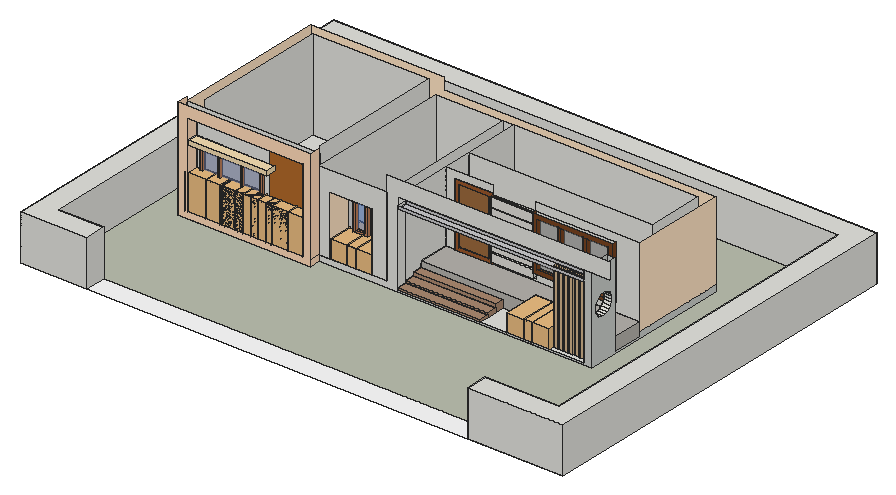
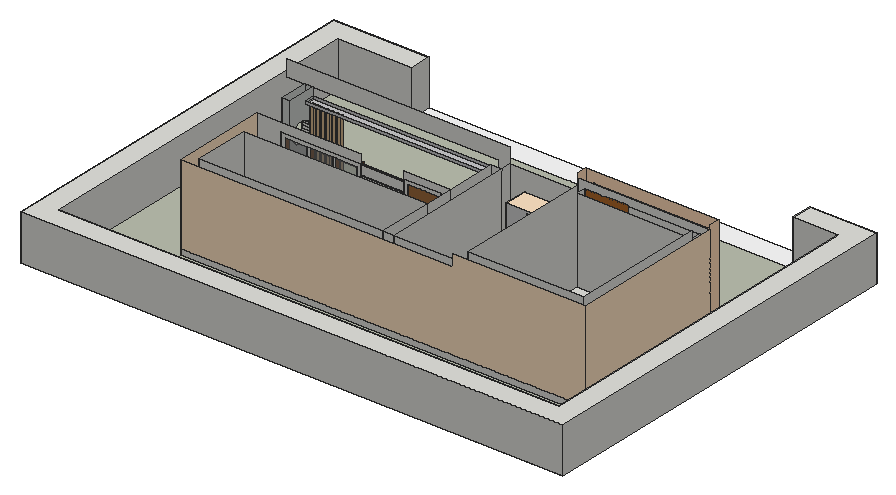
# SketchUp Ruby script. Lengths in inches.
U = 1.inch
M = Sketchup.active_model
def pt(a) = Geom::Point3d.new(a.map { |v| v * U })
def face(e, loops, mat)
  f = e.add_face(loops[0].map { |a| pt(a) })
  loops[1..].each { |l| e.add_face(l.map { |a| pt(a) }).erase! }
  f.material = f.back_material = mat if mat
  f
end
# faces: each face lists its corners as indices into pts; further lists are holes
def faces(e, pts, list, mat = nil) = list.each { |f| face(e, (f[0].is_a?(Array) ? f : [f]).map { |l| l.map { |i| pts[i] } }, mat) }
# xy, xz, yz: faces in a plane at the given z, y or x. An outline is a flat list of corners, or four numbers for a rectangle; further outlines are holes
def ring(l) = l.size == 4 ? [[l[0], l[1]], [l[2], l[1]], [l[2], l[3]], [l[0], l[3]]] : l.each_slice(2).to_a
def flat(e, list, mat, &to3) = list.each { |f| face(e, (f[0].is_a?(Array) ? f : [f]).map { |l| ring(l).map { |u, v| to3.(u, v) } }, mat) }
def xy(e, z, list, mat = nil) = flat(e, list, mat) { |x, y| [x, y, z] }
def xz(e, y, list, mat = nil) = flat(e, list, mat) { |x, z| [x, y, z] }
def yz(e, x, list, mat = nil) = flat(e, list, mat) { |y, z| [x, y, z] }
def lines(e, pts, list) = list.each { |a, b| e.add_line(pt(pts[a]), pt(pts[b])) }
# prism: a flat outline (further loops are holes) pulled along v
def prism(e, loops, v, mat = nil)
  f = face(e, loops, mat); d = Geom::Vector3d.new(v.map { |x| x * U })
  f.pushpull(f.normal.samedirection?(d) ? d.length : -d.length)
end
def box(e, o, s, mat = nil) = prism(e, [[o, [o[0] + s[0], o[1], o[2]], [o[0] + s[0], o[1] + s[1], o[2]], [o[0], o[1] + s[1], o[2]]]], [0, 0, s[2]], mat)
def at(x, y, z, deg = 0) = Geom::Transformation.translation(pt([x, y, z])) * Geom::Transformation.rotation(ORIGIN, Z_AXIS, deg.degrees)
def axes(o, x, y, z) = Geom::Transformation.new([*x, 0, *y, 0, *z, 0, *pt(o).to_a, 1])
def part(name) = M.definitions.add(name)
# library, detail: a bought-in or finely detailed component or shape, given as its bounding box
def library(name, o, s) = part(name).tap { |d| box(d.entities, o, s) }
def detail(e, o, s) = box(e.add_group.entities, o, s)
def put(e, d, t, mat = nil) = e.add_instance(d, t).tap { |i| i.material = mat if mat }
def group(e, t, mat = nil) = e.add_group.tap { |g| g.transformation = t; g.material = mat if mat }.entities
root = M.entities
M.materials.add("[0012_Bisque]").color = [255, 228, 196]
M.materials.add("[0027_PeachPuff]").color = [255, 218, 185]
M.materials.add("[0034_Wheat]").color = [245, 222, 179]
M.materials.add("[0035_Tan]").color = [210, 180, 140]
M.materials.add("[Basic Tile]").color = [203, 206, 202]
M.materials.add("[Cladding Siding White]").color = [207, 207, 207]
M.materials.add("[Color M00]").color = [255, 255, 255]
M.materials.add("[Pavers with Grass Brick]").color = [187, 192, 176]
M.materials.add("[Polished Concrete New]").color = [200, 200, 203]
M.materials.add("[Terrazzo Tile Accent]").color = [224, 221, 217]
M.materials.add("[Tile Travertine 2 inch]").color = [181, 178, 172]
M.materials.add("[Tile Veriegated Stone]").color = [171, 137, 112]
M.materials.add("[Translucent Glass Blue]").color = [100, 149, 237]
M.materials["[Translucent Glass Blue]"].alpha = 0.5
M.materials.add("[Translucent Glass Gray]").color = [128, 128, 128]
M.materials["[Translucent Glass Gray]"].alpha = 0.5
M.materials.add("[Translucent Glass Sky Reflection]").color = [126, 138, 183]
M.materials["[Translucent Glass Sky Reflection]"].alpha = 0.52
M.materials.add("[Wood Bamboo]").color = [177, 105, 43]
M.materials.add("[Wood Cherry Original]").color = [119, 67, 33]
M.materials.add("[Wood Cherry Original]1").color = [152, 86, 42]
M.materials.add("[Wood Floor]").color = [155, 105, 61]
M.materials.add("[Wood Veneer 02]").color = [190, 128, 91]
c1 = library("Flora+17",[-57.52,158.6,-38.64],[66.99,62.88,77.28])
c2 = library("chau cay",[-24.34,-109.24,0],[56.46,62.58,79.69])
xy(root,0,[[0,0,0,591.67,820.1875,591.67,820.1875,0,676.89,0,676.89,32.2,787.99,32.2,787.99,559.47,32.2,559.47,32.2,32.2,99.92,32.2,99.92,0],[72.24,206.91,272.73,223.85],[72.24,223.85,684.44,458.94]])
xy(root,0,[[99.92,0,676.89,32.2]],"[Color M00]")
xy(root,0,[[[32.2,32.2,787.99,559.47],[72.24,206.91,272.73,223.85]]],"[Pavers with Grass Brick]")
xy(root,2.375,[[391.12,223.85,515.24,238.73],[[515.24,223.85,671.95,268.03],[620.18,231.6,626.53,236.51],[628.05,231.6,634.31,236.51],[660.62,231.6,666.86,236.51],[643.87,231.6,649.89,236.51],[635.99,231.6,641.99,236.51],[652.18,231.6,658.09,236.51]],[620.18,231.6,626.53,236.51],[628.05,231.6,634.31,236.51],[635.99,231.6,641.99,236.51],
  [643.87,231.6,649.89,236.51],[652.18,231.6,658.09,236.51],[660.62,231.6,666.86,236.51],[391.12,238.73,515.24,253.38],[391.12,253.38,515.24,268.03]])
xy(root,5.8125,[[391.12,223.85,515.24,238.73]],"[Tile Veriegated Stone]")
xy(root,9,[[87.11,223.85,261.95,238.73],[272.73,223.85,272.73,444.0625,374.48,444.0625,374.48,223.85,352.6,223.85,352.6,259.48,287.9,259.48,287.9,223.85],[87.11,238.73,261.95,444.0625],[374.48,238.73,391.12,444.0625],[391.12,358.92,668.6875,444.0625]])
xy(root,9,[[287.9,223.85,352.6,259.48]],"[0012_Bisque]")
xy(root,9,[[87.11,206.91,261.95,223.85]],"[0027_PeachPuff]")
xy(root,9,[[391.12,238.73,515.24,253.38]],"[Tile Veriegated Stone]")
xy(root,14,[[391.12,253.38,515.24,268.03]],"[Tile Veriegated Stone]")
xy(root,22.51,[[406.1,313.78,461.1,315.41]])
xy(root,22.51,[[391.12,268.03,684.44,268.03,684.44,315.41,461.1,315.41,461.1,313.78,406.1,313.78,406.1,315.41,391.12,315.41]],"[Tile Travertine 2 inch]")
xy(root,26.45,[[461.1,311.53,526.2,315.41]],"[Terrazzo Tile Accent]")
xy(root,27.37,[[410.96,313.78,456.24,315.41]],"[Wood Cherry Original]1")
xy(root,34.36,[[298.82,254.6,320.82,259.48]],"[Wood Veneer 02]")
xy(root,34.89,[[526.2,309.72,646.95,315.41]])
xy(root,38.29,[[302.75,254.6,316.89,259.48]],"[Wood Veneer 02]")
xy(root,39.1875,[[461.1,311.53,526.2,315.41]])
xy(root,41.13,[[564.27,309.72,569.69,315.41],[602.52,309.72,607.94,315.41]])
xy(root,41.13,[[532.4375,309.72,564.27,315.41],[569.69,309.72,602.52,315.41],[607.94,309.72,640.71,315.41]],"[Wood Cherry Original]")
xy(root,41.89,[[461.1,311.53,526.2,315.41]],"[Terrazzo Tile Accent]")
xy(root,44.5,[[94.34,221.35,188.94,223.85]])
xy(root,48.77,[[121.4,221.35,124.96,223.85],[155.64,221.35,158.77,223.85]])
xy(root,48.77,[[98.6,221.35,121.4,223.85],[124.96,221.35,155.64,223.85],[158.77,221.35,184.67,223.85]],"[Wood Veneer 02]")
xy(root,54.625,[[461.1,311.53,526.2,315.41]])
xy(root,56.76,[[461.1,311.53,526.2,315.41]],"[Terrazzo Tile Accent]")
xy(root,69.1875,[[0,0,99.92,0,99.92,32.2,32.2,32.2,32.2,559.47,787.99,559.47,787.99,32.2,676.89,32.2,676.89,0,820.1875,0,820.1875,591.67,0,591.67]])
xy(root,69.5,[[461.1,311.53,526.2,315.41]])
xy(root,71.64,[[461.1,311.53,526.2,315.41]],"[Terrazzo Tile Accent]")
xy(root,84.375,[[461.1,311.53,526.2,315.41]])
xy(root,86.51,[[461.1,311.53,526.2,315.41]],"[Terrazzo Tile Accent]")
xy(root,92.31,[[302.75,254.6,316.89,259.48]])
xy(root,93.36,[[121.4,221.35,124.96,223.85],[155.64,221.35,158.77,223.85]])
xy(root,93.36,[[98.6,221.35,121.4,223.85],[124.96,221.35,155.64,223.85],[158.77,221.35,184.67,223.85]],"[Wood Veneer 02]")
xy(root,96.24,[[298.82,254.6,320.82,259.48]],"[Wood Veneer 02]")
xy(root,97.625,[[94.34,221.35,188.94,223.85]])
xy(root,99.25,[[461.1,311.53,526.2,315.41]])
xy(root,99.28,[[287.9,223.85,352.6,259.48]],"[0012_Bisque]")
xy(root,99.28,[[87.11,207.66,205.99,223.85]],"[0034_Wheat]")
xy(root,101.39,[[461.1,311.53,526.2,315.41]],"[Terrazzo Tile Accent]")
xy(root,105.41,[[87.11,207.66,205.99,223.85]],"[0034_Wheat]")
xy(root,110.47,[[564.27,309.72,569.69,315.41],[602.52,309.72,607.94,315.41]])
xy(root,110.47,[[532.4375,309.72,564.27,315.41],[569.69,309.72,602.52,315.41],[607.94,309.72,640.71,315.41]],"[Wood Cherry Original]")
xy(root,112.27,[[[391.12,223.85,671.95,238.73],[620.18,231.6,626.53,236.51],[628.05,231.6,634.31,236.51],[660.62,231.6,666.86,236.51],[643.87,231.6,649.89,236.51],[635.99,231.6,641.99,236.51],[652.18,231.6,658.09,236.51]]],"[Polished Concrete New]")
xy(root,113.71,[[410.96,313.78,456.24,315.41]],"[Wood Cherry Original]1")
xy(root,114.125,[[461.1,311.53,526.2,315.41]])
xz(root,0,[[0,0,99.92,69.1875],[676.89,0,820.1875,69.1875]])
xz(root,32.2,[[32.2,0,99.92,69.1875],[676.89,0,787.99,69.1875]])
xz(root,206.91,[[[72.24,0,272.73,152.4375],[87.11,9,261.95,135.55]]],"[0027_PeachPuff]")
xz(root,207.66,[[87.11,99.28,205.99,105.41]],"[0034_Wheat]")
xz(root,221.35,[[[94.34,44.5,188.94,97.625],[98.6,48.77,184.67,93.36]],[121.4,48.77,124.96,93.36],[155.64,48.77,158.77,93.36]],"[Wood Veneer 02]")
xz(root,223.85,[[[72.24,0,272.73,146.125],[87.11,9,261.95,135.55]],[272.73,0,391.12,0,391.12,129,711.13,129,711.13,152.4375,374.48,152.4375,374.48,9,272.73,9],[[87.11,9,196.88,99.28],[94.34,44.5,188.94,97.625]],[272.73,9,287.9,9,287.9,99.28,352.6,99.28,352.6,9,374.48,9,374.48,129,272.73,129],[[94.34,44.5,188.94,97.625],[98.6,48.77,184.67,93.36]],
  [121.4,48.77,124.96,93.36],[155.64,48.77,158.77,93.36],[87.11,99.28,196.88,105.41],[196.88,99.28,205.99,105.41],[87.11,105.41,196.88,135.55]])
xz(root,223.85,[[391.12,0,684.44,0,684.44,129,671.95,129,671.95,2.375,391.12,2.375]],"[Basic Tile]")
xz(root,223.85,[[391.12,112.27,671.95,116.34]],"[Polished Concrete New]")
xz(root,223.85,[[391.12,2.375,515.24,5.8125]],"[Tile Veriegated Stone]")
xz(root,223.85,[[98.6,48.77,121.4,93.36],[124.96,48.77,155.64,93.36],[158.77,48.77,184.67,93.36]],"[Translucent Glass Sky Reflection]")
xz(root,223.85,[[196.88,9,261.95,9,261.95,135.55,196.88,135.55,196.88,105.41,205.99,105.41,205.99,99.28,196.88,99.28]],"[Wood Bamboo]")
xz(root,231.6,[[620.18,2.375,626.53,112.27],[628.05,2.375,634.31,112.27],[635.99,2.375,641.99,112.27],[643.87,2.375,649.89,112.27],[652.18,2.375,658.09,112.27],
  [660.62,2.375,666.86,112.27]],"[0035_Tan]")
xz(root,236.51,[[620.18,2.375,626.53,112.27],[628.05,2.375,634.31,112.27],[635.99,2.375,641.99,112.27],[643.87,2.375,649.89,112.27],[652.18,2.375,658.09,112.27],
  [660.62,2.375,666.86,112.27]],"[0035_Tan]")
xz(root,238.73,[[391.12,2.375,515.24,5.8125],[87.11,9,261.95,135.55],[374.48,9,391.12,129]])
xz(root,238.73,[[391.12,112.27,671.95,116.34]],"[Polished Concrete New]")
xz(root,238.73,[[391.12,5.8125,515.24,9]],"[Tile Veriegated Stone]")
xz(root,253.38,[[391.12,2.375,515.24,9]])
xz(root,253.38,[[391.12,9,515.24,14]],"[Tile Veriegated Stone]")
xz(root,254.6,[[[298.82,34.36,320.82,96.24],[302.75,38.29,316.89,92.31]]],"[Wood Veneer 02]")
xz(root,259.48,[[[298.82,34.36,320.82,96.24],[302.75,38.29,316.89,92.31]]])
xz(root,259.48,[[[287.9,9,352.6,99.28],[298.82,34.36,320.82,96.24]]],"[Cladding Siding White]")
xz(root,259.48,[[302.75,38.29,316.89,92.31]],"[Translucent Glass Blue]")
xz(root,268.03,[[391.12,2.375,515.24,14]])
xz(root,268.03,[[671.95,22.51,684.44,129]],"[Basic Tile]")
xz(root,268.03,[[515.24,2.375,671.95,2.375,671.95,22.51,391.12,22.51,391.12,14,515.24,14]],"[Tile Travertine 2 inch]")
xz(root,309.72,[[[526.2,34.89,646.95,116.71],[532.4375,41.13,640.71,110.47]],[564.27,41.13,569.69,110.47],[602.52,41.13,607.94,110.47]],"[Wood Cherry Original]")
xz(root,311.53,[[461.1,26.45,526.2,39.1875],[461.1,41.89,526.2,54.625],[461.1,56.76,526.2,69.5],[461.1,71.64,526.2,84.375],[461.1,86.51,526.2,99.25],
  [461.1,101.39,526.2,114.125]],"[Terrazzo Tile Accent]")
xz(root,313.78,[[[406.1,22.51,461.1,118.57],[410.96,27.37,456.24,113.71]]],"[Wood Cherry Original]1")
xz(root,315.41,[[391.12,2.375,684.44,22.51],[391.12,22.51,406.1,22.51,406.1,118.57,461.1,118.57,461.1,129,391.12,129],[[406.1,22.51,461.1,118.57],[410.96,27.37,456.24,113.71]],[461.1,22.51,526.2,26.45],[526.2,22.51,684.44,22.51,684.44,129,526.2,129,526.2,116.71,646.95,116.71,646.95,34.89,526.2,34.89],
  [461.1,26.45,526.2,39.1875],[[526.2,34.89,646.95,116.71],[532.4375,41.13,640.71,110.47]],[461.1,39.1875,526.2,41.89],[564.27,41.13,569.69,110.47],[602.52,41.13,607.94,110.47],
  [461.1,41.89,526.2,54.625],[461.1,54.625,526.2,56.76],[461.1,56.76,526.2,69.5],[461.1,69.5,526.2,71.64],[461.1,71.64,526.2,84.375],
  [461.1,84.375,526.2,86.51],[461.1,86.51,526.2,99.25],[461.1,99.25,526.2,101.39],[461.1,101.39,526.2,114.125],[461.1,114.125,526.2,116.26]])
xz(root,315.41,[[532.4375,41.13,564.27,110.47],[569.69,41.13,602.52,110.47],[607.94,41.13,640.71,110.47]],"[Translucent Glass Gray]")
xz(root,315.41,[[410.96,27.37,456.24,113.71]],"[Wood Floor]")
xz(root,358.92,[[391.12,9,668.6875,129]])
xz(root,444.0625,[[87.11,9,261.95,146.125],[272.73,9,374.48,129],[374.48,9,391.12,129],[391.12,9,668.6875,129]])
xz(root,458.94,[[72.24,0,684.44,9]])
xz(root,458.94,[[72.24,9,72.24,146.125,272.73,146.125,272.73,129,684.44,129,684.44,9]],"[0012_Bisque]")
xz(root,559.47,[[32.2,0,787.99,69.1875]])
xz(root,591.67,[[0,0,820.1875,69.1875]])
yz(root,0,[[0,0,591.67,69.1875]])
yz(root,32.2,[[32.2,0,559.47,69.1875]])
yz(root,72.24,[[223.85,0,458.94,9]])
yz(root,72.24,[[223.85,9,458.94,146.125]],"[0012_Bisque]")
yz(root,72.24,[[206.91,0,223.85,9],[206.91,9,223.85,152.4375]],"[0027_PeachPuff]")
yz(root,87.11,[[223.85,9,238.73,135.55],[238.73,9,444.0625,146.125],[207.66,99.28,223.85,105.41]])
yz(root,87.11,[[206.91,9,223.85,9,223.85,99.28,207.66,99.28,207.66,105.41,223.85,105.41,223.85,135.55,206.91,135.55]],"[0027_PeachPuff]")
yz(root,94.34,[[221.35,44.5,223.85,97.625]],"[Wood Veneer 02]")
yz(root,98.6,[[221.35,48.77,223.85,93.36]],"[Wood Veneer 02]")
yz(root,99.92,[[0,0,32.2,69.1875]])
yz(root,121.4,[[221.35,48.77,223.85,93.36]],"[Wood Veneer 02]")
yz(root,124.96,[[221.35,48.77,223.85,93.36]],"[Wood Veneer 02]")
yz(root,155.64,[[221.35,48.77,223.85,93.36]],"[Wood Veneer 02]")
yz(root,158.77,[[221.35,48.77,223.85,93.36]],"[Wood Veneer 02]")
yz(root,184.67,[[221.35,48.77,223.85,93.36]],"[Wood Veneer 02]")
yz(root,188.94,[[221.35,44.5,223.85,97.625]],"[Wood Veneer 02]")
yz(root,205.99,[[207.66,99.28,223.85,105.41]],"[0034_Wheat]")
yz(root,261.95,[[223.85,9,238.73,135.55],[238.73,9,444.0625,146.125]])
yz(root,261.95,[[206.91,9,223.85,135.55]],"[0027_PeachPuff]")
yz(root,272.73,[[223.85,9,444.0625,129]])
yz(root,272.73,[[206.91,0,223.85,9],[206.91,9,223.85,152.4375]],"[0027_PeachPuff]")
yz(root,287.9,[[223.85,9,259.48,99.28]],"[0012_Bisque]")
yz(root,298.82,[[254.6,34.36,259.48,96.24]],"[Wood Veneer 02]")
yz(root,302.75,[[254.6,38.29,259.48,92.31]],"[Wood Veneer 02]")
yz(root,316.89,[[254.6,38.29,259.48,92.31]],"[Wood Veneer 02]")
yz(root,320.82,[[254.6,34.36,259.48,96.24]],"[Wood Veneer 02]")
yz(root,352.6,[[223.85,9,259.48,99.28]],"[0012_Bisque]")
yz(root,374.48,[[223.85,9,238.73,129],[238.73,9,444.0625,129]])
yz(root,391.12,[[223.85,2.375,238.73,5.8125],[238.73,2.375,253.38,9],[253.38,2.375,268.03,9],[268.03,2.375,315.41,9],[223.85,5.8125,238.73,112.27],
  [238.73,9,253.38,9,253.38,14,268.03,14,268.03,22.51,315.41,22.51,315.41,129,238.73,129],[253.38,9,268.03,14],[268.03,9,315.41,22.51],[315.41,9,358.92,129],[358.92,9,444.0625,129],
  [223.85,112.27,238.73,116.34]])
yz(root,406.1,[[313.78,22.51,315.41,118.57]],"[Wood Floor]")
yz(root,410.96,[[313.78,27.37,315.41,113.71]],"[Wood Cherry Original]1")
yz(root,456.24,[[313.78,27.37,315.41,113.71]],"[Wood Cherry Original]1")
yz(root,461.1,[[313.78,26.45,315.41,28.76],[313.78,28.76,315.41,39.1875],[313.78,41.89,315.41,44.2],[313.78,44.2,315.41,54.625],[313.78,56.76,315.41,59.07],
  [313.78,59.07,315.41,69.5],[313.78,71.64,315.41,73.95],[313.78,73.95,315.41,84.375],[313.78,86.51,315.41,88.82],[313.78,88.82,315.41,99.25],
  [313.78,101.39,315.41,103.7],[313.78,103.7,315.41,114.125]])
yz(root,461.1,[[311.53,26.45,313.78,39.1875],[311.53,41.89,313.78,54.625],[311.53,56.76,313.78,69.5],[311.53,71.64,313.78,84.375],[311.53,86.51,313.78,99.25],
  [311.53,101.39,313.78,114.125]],"[Terrazzo Tile Accent]")
yz(root,461.1,[[313.78,22.51,315.41,26.45],[313.78,39.1875,315.41,41.89],[313.78,54.625,315.41,56.76],[313.78,69.5,315.41,71.64],[313.78,84.375,315.41,86.51],
  [313.78,99.25,315.41,101.39],[313.78,114.125,315.41,116.26]],"[Wood Cherry Original]1")
yz(root,515.24,[[223.85,2.375,238.73,5.8125],[238.73,2.375,253.38,9],[253.38,2.375,268.03,14]],"[Tile Veriegated Stone]")
yz(root,526.2,[[311.53,26.45,315.41,26.89],[311.53,26.89,315.41,34.89],[311.53,34.89,315.41,39.1875],[311.53,41.89,315.41,42.33],[311.53,42.33,315.41,54.625],
  [311.53,56.76,315.41,57.21],[311.53,57.21,315.41,69.5],[311.53,71.64,315.41,72.08],[311.53,72.08,315.41,84.375],[311.53,86.51,315.41,86.96],
  [311.53,86.96,315.41,99.25],[311.53,101.39,315.41,101.83],[311.53,101.83,315.41,114.125]])
yz(root,526.2,[[309.72,34.89,309.72,116.71,311.53,116.71,311.53,116.26,315.41,116.26,315.41,114.125,311.53,114.125,311.53,101.39,315.41,101.39,315.41,99.25,311.53,99.25,311.53,86.51,315.41,86.51,315.41,84.375,311.53,84.375,311.53,71.64,315.41,71.64,315.41,69.5,311.53,69.5,311.53,56.76,315.41,56.76,315.41,54.625,311.53,54.625,311.53,41.89,315.41,41.89,315.41,39.1875,311.53,39.1875,311.53,34.89]],"[Wood Cherry Original]")
yz(root,532.4375,[[309.72,41.13,315.41,110.47]],"[Wood Cherry Original]")
yz(root,564.27,[[309.72,41.13,315.41,110.47]],"[Wood Cherry Original]")
yz(root,569.69,[[309.72,41.13,315.41,110.47]],"[Wood Cherry Original]")
yz(root,602.52,[[309.72,41.13,315.41,110.47]],"[Wood Cherry Original]")
yz(root,607.94,[[309.72,41.13,315.41,110.47]],"[Wood Cherry Original]")
yz(root,620.18,[[231.6,2.375,236.51,112.27]],"[0035_Tan]")
yz(root,626.53,[[231.6,2.375,236.51,112.27]],"[0035_Tan]")
yz(root,628.05,[[231.6,2.375,236.51,112.27]],"[0035_Tan]")
yz(root,634.31,[[231.6,2.375,236.51,112.27]],"[0035_Tan]")
yz(root,635.99,[[231.6,2.375,236.51,112.27]],"[0035_Tan]")
yz(root,640.71,[[309.72,41.13,315.41,110.47]],"[Wood Cherry Original]")
yz(root,641.99,[[231.6,2.375,236.51,112.27]],"[0035_Tan]")
yz(root,643.87,[[231.6,2.375,236.51,112.27]],"[0035_Tan]")
yz(root,646.95,[[309.72,34.89,315.41,116.71]],"[Wood Cherry Original]")
yz(root,649.89,[[231.6,2.375,236.51,112.27]],"[0035_Tan]")
yz(root,652.18,[[231.6,2.375,236.51,112.27]],"[0035_Tan]")
yz(root,658.09,[[231.6,2.375,236.51,112.27]],"[0035_Tan]")
yz(root,660.62,[[231.6,2.375,236.51,112.27]],"[0035_Tan]")
yz(root,666.86,[[231.6,2.375,236.51,112.27]],"[0035_Tan]")
yz(root,668.6875,[[358.92,9,444.0625,129]])
yz(root,671.95,[[[223.85,2.375,223.85,112.27,238.73,112.27,238.73,116.34,223.85,116.34,223.85,129,268.03,129,268.03,2.375],[245.94,60.87,250.06,61.41,253.91,63.01,257.21,65.54,259.74,68.84,261.33,72.68,261.88,76.81,261.33,80.93,259.74,84.78,257.21,88.08,253.91,90.61,250.06,92.2,245.94,92.75,241.82,92.2,238.73,90.92,237.97,90.61,234.67,88.08,232.14,84.78,230.55,80.93,230,76.81,230.55,72.68,232.14,68.84,234.67,65.54,237.97,63.01,238.73,62.69,241.82,61.41]]],"[Basic Tile]")
yz(root,676.89,[[0,0,32.2,69.1875]])
yz(root,684.44,[[315.41,9,458.94,129]],"[0012_Bisque]")
yz(root,684.44,[[[223.85,0,458.94,0,458.94,9,315.41,9,315.41,2.375,268.03,2.375,268.03,129,223.85,129],[245.94,60.87,241.82,61.41,237.97,63.01,234.67,65.54,232.14,68.84,230.55,72.68,230,76.81,230.55,80.93,232.14,84.78,234.67,88.08,237.97,90.61,241.82,92.2,245.94,92.75,250.06,92.2,253.91,90.61,257.21,88.08,259.74,84.78,261.33,80.93,261.88,76.81,261.33,72.68,259.74,68.84,257.21,65.54,253.91,63.01,250.06,61.41]]],"[Basic Tile]")
yz(root,684.44,[[268.03,2.375,315.41,22.51]],"[Tile Travertine 2 inch]")
yz(root,787.99,[[32.2,0,559.47,69.1875]])
yz(root,820.1875,[[0,0,591.67,69.1875]])
p = [[671.95,245.94,60.87],[671.95,241.82,61.41],[684.44,241.82,61.41],[684.44,245.94,60.87],[671.95,250.06,61.41],[684.44,250.06,61.41],
  [671.95,238.73,62.69],[671.95,237.97,63.01],[684.44,237.97,63.01],[671.95,253.91,63.01],[684.44,253.91,63.01],[671.95,234.67,65.54],
  [684.44,234.67,65.54],[671.95,257.21,65.54],[684.44,257.21,65.54],[671.95,232.14,68.84],[684.44,232.14,68.84],[671.95,259.74,68.84],
  [684.44,259.74,68.84],[671.95,230.55,72.68],[684.44,230.55,72.68],[671.95,261.33,72.68],[684.44,261.33,72.68],[671.95,230,76.81],
  [684.44,230,76.81],[671.95,261.88,76.81],[684.44,261.88,76.81],[671.95,230.55,80.93],[684.44,230.55,80.93],[671.95,261.33,80.93],
  [684.44,261.33,80.93],[671.95,232.14,84.78],[684.44,232.14,84.78],[671.95,259.74,84.78],[684.44,259.74,84.78],[671.95,234.67,88.08],
  [684.44,234.67,88.08],[671.95,257.21,88.08],[684.44,257.21,88.08],[671.95,237.97,90.61],[684.44,237.97,90.61],[671.95,253.91,90.61],
  [684.44,253.91,90.61],[671.95,238.73,90.92],[671.95,241.82,92.2],[684.44,241.82,92.2],[671.95,250.06,92.2],[684.44,250.06,92.2],
  [671.95,245.94,92.75],[684.44,245.94,92.75],[668.6875,358.92,9],[668.6875,315.41,9],[261.95,444.0625,9],[272.73,444.0625,9]]
faces(root,p,[[0,1,2,3],[4,0,3,5],[6,7,8,2,1],[9,4,5,10],[7,11,12,8],[13,9,10,14],[11,15,16,12],[17,13,14,18],
  [15,19,20,16],[21,17,18,22],[19,23,24,20],[25,21,22,26],[23,27,28,24],[29,25,26,30],[27,31,32,28],[33,29,30,34],
  [31,35,36,32],[37,33,34,38],[35,39,40,36],[41,37,38,42],[43,44,45,40,39],[46,41,42,47],[44,48,49,45],[48,46,47,49]])
lines(root,p,[[50,51],[52,53]])
put(root,c1,axes([614.65,85.87,16.06],[0.57,0,0],[0,0.87,0],[0,0,0.3541]))
put(root,c1,axes([588.19,85.87,16.06],[0.57,0,0],[0,0.87,0],[0,0,0.3541]))
put(root,c2,axes([107.16,241.87,9],[1,0,0],[0,0.32,0],[0,0,0.66972]))
put(root,c2,axes([139.16,241.87,9],[1,0,0],[0,0.32,0],[0,0,0.66972]))
put(root,c2,axes([160.85,241.87,9],[1,0,0],[0,0.32,0],[0,0,0.66972]))
put(root,c2,axes([182.91,241.87,9],[1,0,0],[0,0.32,0],[0,0,0.66972]))
put(root,c2,axes([229.83,241.87,9],[1,0,0],[0,0.32,0],[0,0,0.66972]))
put(root,c2,axes([207.02,241.87,9],[1,0,0],[0,0.32,0],[0,0,0.66972]))
put(root,c1,axes([347.2,85.87,22.68],[0.57,0,0],[0,0.87,0],[0,0,0.3541]))
put(root,c1,axes([323.2,85.87,22.68],[0.57,0,0],[0,0.87,0],[0,0,0.3541]))
